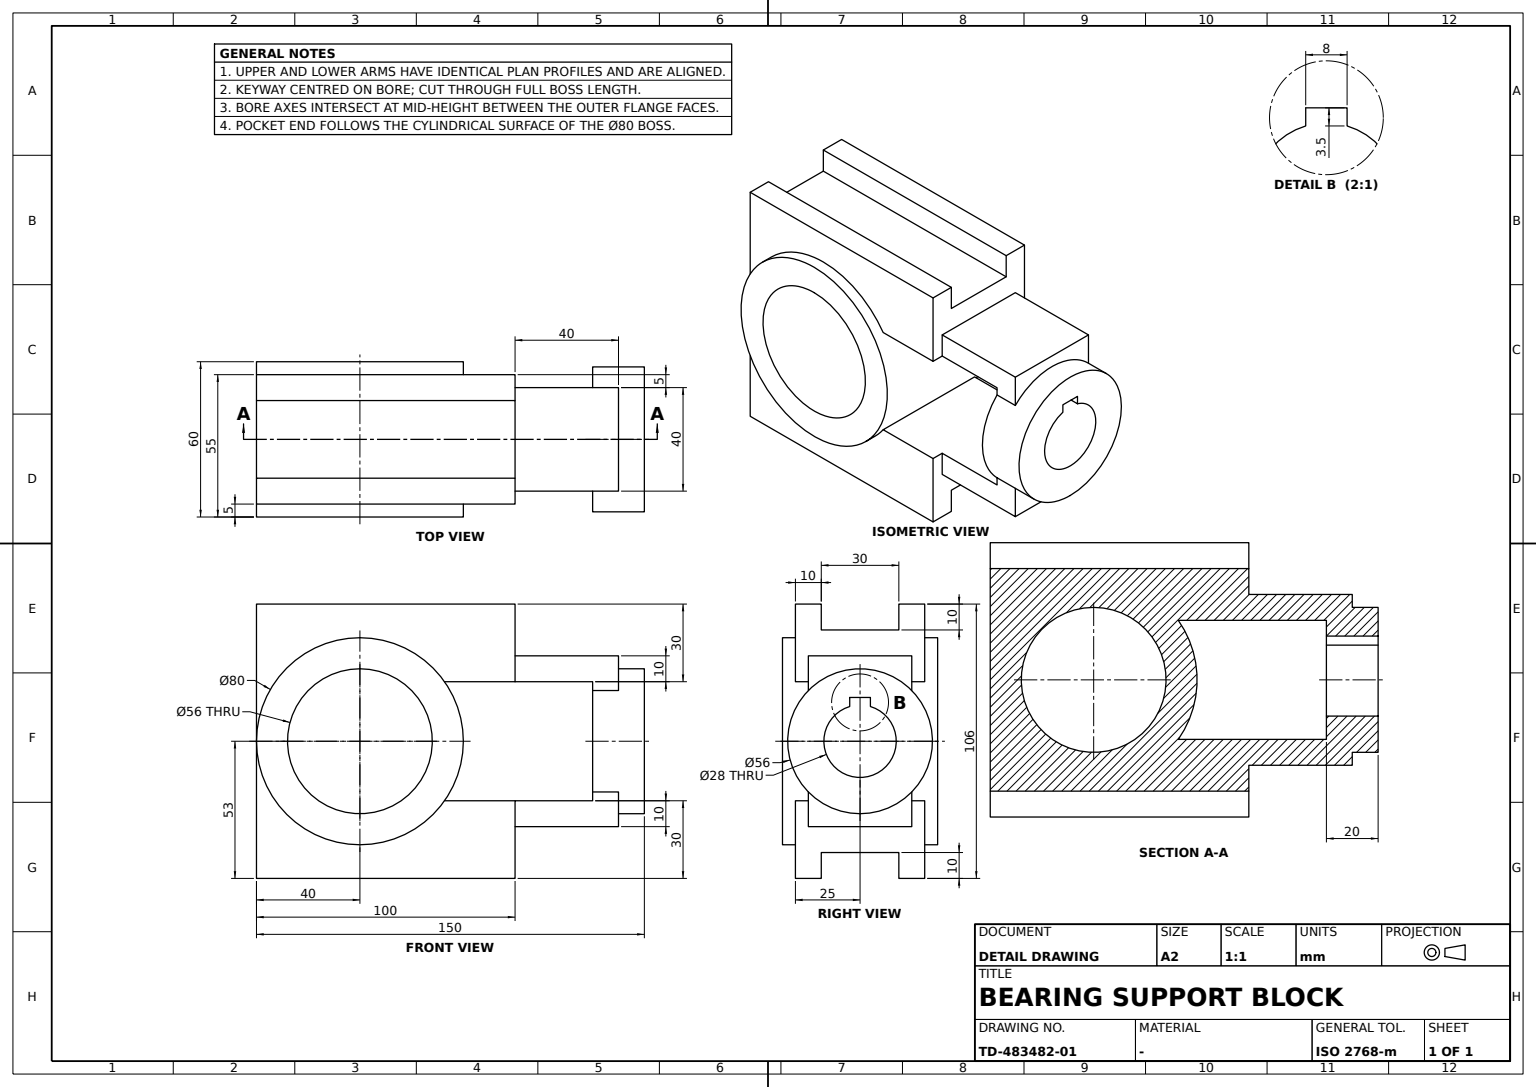
ISO-10303-21;
HEADER;
FILE_DESCRIPTION((''),'2;1');
FILE_NAME('','',(''),(''),'','','');
FILE_SCHEMA(('AUTOMOTIVE_DESIGN'));
ENDSEC;
DATA;
#1=APPLICATION_CONTEXT('');
#2=PRODUCT_CONTEXT('',#1,'mechanical');
#3=PRODUCT('','','',(#2));
#4=PRODUCT_DEFINITION_FORMATION('','',#3);
#5=PRODUCT_DEFINITION_CONTEXT('',#1,'design');
#6=PRODUCT_DEFINITION('','',#4,#5);
#7=PRODUCT_DEFINITION_SHAPE('','',#6);
#8=(LENGTH_UNIT()NAMED_UNIT(*)SI_UNIT(.MILLI.,.METRE.));
#9=(NAMED_UNIT(*)PLANE_ANGLE_UNIT()SI_UNIT($,.RADIAN.));
#10=(NAMED_UNIT(*)SI_UNIT($,.STERADIAN.)SOLID_ANGLE_UNIT());
#11=UNCERTAINTY_MEASURE_WITH_UNIT(LENGTH_MEASURE(0.005),#8,'distance_accuracy_value','');
#12=(GEOMETRIC_REPRESENTATION_CONTEXT(3)GLOBAL_UNCERTAINTY_ASSIGNED_CONTEXT((#11))GLOBAL_UNIT_ASSIGNED_CONTEXT((#8,#9,#10))REPRESENTATION_CONTEXT('',''));
#13=CARTESIAN_POINT('',(40.,-30.,81.));
#14=VERTEX_POINT('',#13);
#15=CARTESIAN_POINT('',(40.,-30.,53.));
#16=DIRECTION('',(0.,1.,0.));
#17=DIRECTION('',(0.,0.,1.));
#18=AXIS2_PLACEMENT_3D('',#15,#16,#17);
#19=CIRCLE('',#18,28.);
#20=EDGE_CURVE('',#14,#14,#19,.T.);
#21=ORIENTED_EDGE('',*,*,#20,.F.);
#22=EDGE_LOOP('',(#21));
#23=FACE_BOUND('',#22,.T.);
#24=CARTESIAN_POINT('',(40.,30.,81.));
#25=VERTEX_POINT('',#24);
#26=CARTESIAN_POINT('',(40.,30.,53.));
#27=AXIS2_PLACEMENT_3D('',#26,#16,#17);
#28=CIRCLE('',#27,28.);
#29=EDGE_CURVE('',#25,#25,#28,.T.);
#30=ORIENTED_EDGE('',*,*,#29,.T.);
#31=EDGE_LOOP('',(#30));
#32=FACE_BOUND('',#31,.T.);
#33=CARTESIAN_POINT('',(40.,29.9,53.));
#34=DIRECTION('',(0.,-1.,0.));
#35=DIRECTION('',(1.,0.,0.));
#36=AXIS2_PLACEMENT_3D('',#33,#34,#35);
#37=CYLINDRICAL_SURFACE('',#36,28.);
#38=ADVANCED_FACE('',(#23,#32),#37,.F.);
#39=CARTESIAN_POINT('',(100.,15.,10.));
#40=VERTEX_POINT('',#39);
#41=CARTESIAN_POINT('',(100.,15.,0.));
#42=VERTEX_POINT('',#41);
#43=CARTESIAN_POINT('',(100.,15.,106.));
#44=DIRECTION('',(0.,0.,-1.));
#45=VECTOR('',#44,1000.);
#46=LINE('',#43,#45);
#47=EDGE_CURVE('',#40,#42,#46,.T.);
#48=ORIENTED_EDGE('',*,*,#47,.F.);
#49=CARTESIAN_POINT('',(0.,15.,10.));
#50=VERTEX_POINT('',#49);
#51=DIRECTION('',(-1.,0.,0.));
#52=VECTOR('',#51,1000.);
#53=LINE('',#39,#52);
#54=EDGE_CURVE('',#40,#50,#53,.T.);
#55=ORIENTED_EDGE('',*,*,#54,.T.);
#56=CARTESIAN_POINT('',(0.,15.,0.));
#57=VERTEX_POINT('',#56);
#58=VECTOR('',#17,1000.);
#59=LINE('',#56,#58);
#60=EDGE_CURVE('',#57,#50,#59,.T.);
#61=ORIENTED_EDGE('',*,*,#60,.F.);
#62=LINE('',#41,#52);
#63=EDGE_CURVE('',#42,#57,#62,.T.);
#64=ORIENTED_EDGE('',*,*,#63,.F.);
#65=EDGE_LOOP('',(#48,#55,#61,#64));
#66=FACE_BOUND('',#65,.T.);
#67=CARTESIAN_POINT('',(100.,15.,96.));
#68=AXIS2_PLACEMENT_3D('',#67,#34,#17);
#69=PLANE('',#68);
#70=ADVANCED_FACE('',(#66),#69,.T.);
#71=CARTESIAN_POINT('',(150.,4.,66.416408));
#72=VERTEX_POINT('',#71);
#73=CARTESIAN_POINT('',(150.,4.,69.916408));
#74=VERTEX_POINT('',#73);
#75=LINE('',#71,#58);
#76=EDGE_CURVE('',#72,#74,#75,.T.);
#77=ORIENTED_EDGE('',*,*,#76,.F.);
#78=CARTESIAN_POINT('',(150.,-4.,66.416408));
#79=VERTEX_POINT('',#78);
#80=CARTESIAN_POINT('',(150.,0.,53.));
#81=AXIS2_PLACEMENT_3D('',#80,#35,#44);
#82=CIRCLE('',#81,14.);
#83=EDGE_CURVE('',#79,#72,#82,.T.);
#84=ORIENTED_EDGE('',*,*,#83,.F.);
#85=CARTESIAN_POINT('',(150.,-4.,69.916408));
#86=VERTEX_POINT('',#85);
#87=LINE('',#85,#45);
#88=EDGE_CURVE('',#86,#79,#87,.T.);
#89=ORIENTED_EDGE('',*,*,#88,.F.);
#90=VECTOR('',#16,1000.);
#91=LINE('',#85,#90);
#92=EDGE_CURVE('',#86,#74,#91,.T.);
#93=ORIENTED_EDGE('',*,*,#92,.T.);
#94=EDGE_LOOP('',(#77,#84,#89,#93));
#95=FACE_BOUND('',#94,.T.);
#96=CARTESIAN_POINT('',(150.,0.,25.));
#97=VERTEX_POINT('',#96);
#98=CIRCLE('',#81,28.);
#99=EDGE_CURVE('',#97,#97,#98,.T.);
#100=ORIENTED_EDGE('',*,*,#99,.T.);
#101=EDGE_LOOP('',(#100));
#102=FACE_BOUND('',#101,.T.);
#103=CARTESIAN_POINT('',(150.,0.,0.));
#104=AXIS2_PLACEMENT_3D('',#103,#35,#16);
#105=PLANE('',#104);
#106=ADVANCED_FACE('',(#95,#102),#105,.T.);
#107=CARTESIAN_POINT('',(40.,30.,93.));
#108=VERTEX_POINT('',#107);
#109=CIRCLE('',#27,40.);
#110=EDGE_CURVE('',#108,#108,#109,.T.);
#111=ORIENTED_EDGE('',*,*,#110,.T.);
#112=EDGE_LOOP('',(#111));
#113=FACE_BOUND('',#112,.T.);
#114=ORIENTED_EDGE('',*,*,#29,.F.);
#115=EDGE_LOOP('',(#114));
#116=FACE_BOUND('',#115,.T.);
#117=CARTESIAN_POINT('',(0.,30.,0.));
#118=AXIS2_PLACEMENT_3D('',#117,#16,#51);
#119=PLANE('',#118);
#120=ADVANCED_FACE('',(#113,#116),#119,.T.);
#121=CARTESIAN_POINT('',(100.,20.,76.));
#122=VERTEX_POINT('',#121);
#123=CARTESIAN_POINT('',(130.,20.,76.));
#124=VERTEX_POINT('',#123);
#125=VECTOR('',#35,1000.);
#126=LINE('',#121,#125);
#127=EDGE_CURVE('',#122,#124,#126,.T.);
#128=ORIENTED_EDGE('',*,*,#127,.F.);
#129=CARTESIAN_POINT('',(100.,20.,86.));
#130=VERTEX_POINT('',#129);
#131=CARTESIAN_POINT('',(100.,20.,106.));
#132=LINE('',#131,#58);
#133=EDGE_CURVE('',#122,#130,#132,.T.);
#134=ORIENTED_EDGE('',*,*,#133,.T.);
#135=CARTESIAN_POINT('',(140.,20.,86.));
#136=VERTEX_POINT('',#135);
#137=LINE('',#129,#125);
#138=EDGE_CURVE('',#130,#136,#137,.T.);
#139=ORIENTED_EDGE('',*,*,#138,.T.);
#140=CARTESIAN_POINT('',(140.,20.,72.595918));
#141=VERTEX_POINT('',#140);
#142=CARTESIAN_POINT('',(140.,20.,76.));
#143=LINE('',#142,#45);
#144=EDGE_CURVE('',#136,#141,#143,.T.);
#145=ORIENTED_EDGE('',*,*,#144,.T.);
#146=CARTESIAN_POINT('',(130.,20.,72.595918));
#147=VERTEX_POINT('',#146);
#148=LINE('',#140,#125);
#149=EDGE_CURVE('',#147,#141,#148,.T.);
#150=ORIENTED_EDGE('',*,*,#149,.F.);
#151=CARTESIAN_POINT('',(130.,20.,30.));
#152=LINE('',#151,#58);
#153=EDGE_CURVE('',#147,#124,#152,.T.);
#154=ORIENTED_EDGE('',*,*,#153,.T.);
#155=EDGE_LOOP('',(#128,#134,#139,#145,#150,#154));
#156=FACE_BOUND('',#155,.T.);
#157=AXIS2_PLACEMENT_3D('',#121,#16,#17);
#158=PLANE('',#157);
#159=ADVANCED_FACE('',(#156),#158,.T.);
#160=CARTESIAN_POINT('',(100.,-20.,86.));
#161=VERTEX_POINT('',#160);
#162=CARTESIAN_POINT('',(140.,-20.,86.));
#163=VERTEX_POINT('',#162);
#164=LINE('',#160,#125);
#165=EDGE_CURVE('',#161,#163,#164,.T.);
#166=ORIENTED_EDGE('',*,*,#165,.F.);
#167=CARTESIAN_POINT('',(100.,-20.,76.));
#168=VERTEX_POINT('',#167);
#169=CARTESIAN_POINT('',(100.,-20.,106.));
#170=LINE('',#169,#45);
#171=EDGE_CURVE('',#161,#168,#170,.T.);
#172=ORIENTED_EDGE('',*,*,#171,.T.);
#173=CARTESIAN_POINT('',(130.,-20.,76.));
#174=VERTEX_POINT('',#173);
#175=LINE('',#167,#125);
#176=EDGE_CURVE('',#168,#174,#175,.T.);
#177=ORIENTED_EDGE('',*,*,#176,.T.);
#178=CARTESIAN_POINT('',(130.,-20.,72.595918));
#179=VERTEX_POINT('',#178);
#180=CARTESIAN_POINT('',(130.,-20.,86.));
#181=LINE('',#180,#58);
#182=EDGE_CURVE('',#179,#174,#181,.T.);
#183=ORIENTED_EDGE('',*,*,#182,.F.);
#184=CARTESIAN_POINT('',(140.,-20.,72.595918));
#185=VERTEX_POINT('',#184);
#186=LINE('',#184,#125);
#187=EDGE_CURVE('',#179,#185,#186,.T.);
#188=ORIENTED_EDGE('',*,*,#187,.T.);
#189=LINE('',#162,#58);
#190=EDGE_CURVE('',#185,#163,#189,.T.);
#191=ORIENTED_EDGE('',*,*,#190,.T.);
#192=EDGE_LOOP('',(#166,#172,#177,#183,#188,#191));
#193=FACE_BOUND('',#192,.T.);
#194=AXIS2_PLACEMENT_3D('',#160,#34,#44);
#195=PLANE('',#194);
#196=ADVANCED_FACE('',(#193),#195,.T.);
#197=CARTESIAN_POINT('',(130.,-4.,69.916408));
#198=VERTEX_POINT('',#197);
#199=CARTESIAN_POINT('',(130.,4.,69.916408));
#200=VERTEX_POINT('',#199);
#201=LINE('',#197,#90);
#202=EDGE_CURVE('',#198,#200,#201,.T.);
#203=ORIENTED_EDGE('',*,*,#202,.T.);
#204=LINE('',#73,#52);
#205=EDGE_CURVE('',#74,#200,#204,.T.);
#206=ORIENTED_EDGE('',*,*,#205,.F.);
#207=ORIENTED_EDGE('',*,*,#92,.F.);
#208=LINE('',#85,#52);
#209=EDGE_CURVE('',#86,#198,#208,.T.);
#210=ORIENTED_EDGE('',*,*,#209,.T.);
#211=EDGE_LOOP('',(#203,#206,#207,#210));
#212=FACE_BOUND('',#211,.T.);
#213=AXIS2_PLACEMENT_3D('',#85,#17,#16);
#214=PLANE('',#213);
#215=ADVANCED_FACE('',(#212),#214,.F.);
#216=CARTESIAN_POINT('',(0.,-25.,106.));
#217=VERTEX_POINT('',#216);
#218=CARTESIAN_POINT('',(100.,-25.,106.));
#219=VERTEX_POINT('',#218);
#220=LINE('',#216,#125);
#221=EDGE_CURVE('',#217,#219,#220,.T.);
#222=ORIENTED_EDGE('',*,*,#221,.T.);
#223=CARTESIAN_POINT('',(100.,-15.,106.));
#224=VERTEX_POINT('',#223);
#225=CARTESIAN_POINT('',(100.,0.,106.));
#226=LINE('',#225,#90);
#227=EDGE_CURVE('',#219,#224,#226,.T.);
#228=ORIENTED_EDGE('',*,*,#227,.T.);
#229=CARTESIAN_POINT('',(0.,-15.,106.));
#230=VERTEX_POINT('',#229);
#231=LINE('',#229,#52);
#232=EDGE_CURVE('',#224,#230,#231,.T.);
#233=ORIENTED_EDGE('',*,*,#232,.T.);
#234=CARTESIAN_POINT('',(0.,0.,106.));
#235=LINE('',#234,#90);
#236=EDGE_CURVE('',#217,#230,#235,.T.);
#237=ORIENTED_EDGE('',*,*,#236,.F.);
#238=EDGE_LOOP('',(#222,#228,#233,#237));
#239=FACE_BOUND('',#238,.T.);
#240=AXIS2_PLACEMENT_3D('',#234,#17,#35);
#241=PLANE('',#240);
#242=ADVANCED_FACE('',(#239),#241,.T.);
#243=CARTESIAN_POINT('',(130.,4.,66.416408));
#244=VERTEX_POINT('',#243);
#245=LINE('',#243,#58);
#246=EDGE_CURVE('',#244,#200,#245,.T.);
#247=ORIENTED_EDGE('',*,*,#246,.F.);
#248=LINE('',#71,#125);
#249=EDGE_CURVE('',#72,#244,#248,.F.);
#250=ORIENTED_EDGE('',*,*,#249,.F.);
#251=ORIENTED_EDGE('',*,*,#76,.T.);
#252=ORIENTED_EDGE('',*,*,#205,.T.);
#253=EDGE_LOOP('',(#247,#250,#251,#252));
#254=FACE_BOUND('',#253,.T.);
#255=AXIS2_PLACEMENT_3D('',#71,#34,#17);
#256=PLANE('',#255);
#257=ADVANCED_FACE('',(#254),#256,.T.);
#258=CARTESIAN_POINT('',(100.,25.,30.));
#259=VERTEX_POINT('',#258);
#260=CARTESIAN_POINT('',(100.,25.,0.));
#261=VERTEX_POINT('',#260);
#262=LINE('',#260,#45);
#263=EDGE_CURVE('',#259,#261,#262,.T.);
#264=ORIENTED_EDGE('',*,*,#263,.T.);
#265=CARTESIAN_POINT('',(0.,25.,0.));
#266=VERTEX_POINT('',#265);
#267=LINE('',#265,#52);
#268=EDGE_CURVE('',#261,#266,#267,.T.);
#269=ORIENTED_EDGE('',*,*,#268,.T.);
#270=CARTESIAN_POINT('',(0.,25.,53.));
#271=VERTEX_POINT('',#270);
#272=LINE('',#265,#58);
#273=EDGE_CURVE('',#266,#271,#272,.T.);
#274=ORIENTED_EDGE('',*,*,#273,.T.);
#275=CARTESIAN_POINT('',(72.726136,25.,30.));
#276=VERTEX_POINT('',#275);
#277=CARTESIAN_POINT('',(40.,25.,53.));
#278=AXIS2_PLACEMENT_3D('',#277,#16,#17);
#279=CIRCLE('',#278,40.);
#280=EDGE_CURVE('',#276,#271,#279,.T.);
#281=ORIENTED_EDGE('',*,*,#280,.F.);
#282=CARTESIAN_POINT('',(0.,25.,30.));
#283=LINE('',#282,#125);
#284=EDGE_CURVE('',#276,#259,#283,.T.);
#285=ORIENTED_EDGE('',*,*,#284,.T.);
#286=EDGE_LOOP('',(#264,#269,#274,#281,#285));
#287=FACE_BOUND('',#286,.T.);
#288=AXIS2_PLACEMENT_3D('',#265,#16,#51);
#289=PLANE('',#288);
#290=ADVANCED_FACE('',(#287),#289,.T.);
#291=CARTESIAN_POINT('',(140.,0.,86.));
#292=LINE('',#291,#90);
#293=EDGE_CURVE('',#163,#136,#292,.T.);
#294=ORIENTED_EDGE('',*,*,#293,.T.);
#295=ORIENTED_EDGE('',*,*,#138,.F.);
#296=CARTESIAN_POINT('',(100.,0.,86.));
#297=LINE('',#296,#90);
#298=EDGE_CURVE('',#161,#130,#297,.T.);
#299=ORIENTED_EDGE('',*,*,#298,.F.);
#300=ORIENTED_EDGE('',*,*,#165,.T.);
#301=EDGE_LOOP('',(#294,#295,#299,#300));
#302=FACE_BOUND('',#301,.T.);
#303=AXIS2_PLACEMENT_3D('',#160,#44,#16);
#304=PLANE('',#303);
#305=ADVANCED_FACE('',(#302),#304,.F.);
#306=CARTESIAN_POINT('',(0.,25.,106.));
#307=VERTEX_POINT('',#306);
#308=CARTESIAN_POINT('',(100.,25.,106.));
#309=VERTEX_POINT('',#308);
#310=LINE('',#306,#125);
#311=EDGE_CURVE('',#307,#309,#310,.T.);
#312=ORIENTED_EDGE('',*,*,#311,.F.);
#313=CARTESIAN_POINT('',(0.,15.,106.));
#314=VERTEX_POINT('',#313);
#315=EDGE_CURVE('',#314,#307,#235,.T.);
#316=ORIENTED_EDGE('',*,*,#315,.F.);
#317=VERTEX_POINT('',#43);
#318=LINE('',#43,#52);
#319=EDGE_CURVE('',#317,#314,#318,.T.);
#320=ORIENTED_EDGE('',*,*,#319,.F.);
#321=EDGE_CURVE('',#317,#309,#226,.T.);
#322=ORIENTED_EDGE('',*,*,#321,.T.);
#323=EDGE_LOOP('',(#312,#316,#320,#322));
#324=FACE_BOUND('',#323,.T.);
#325=ADVANCED_FACE('',(#324),#241,.T.);
#326=ORIENTED_EDGE('',*,*,#249,.T.);
#327=CARTESIAN_POINT('',(130.,-4.,66.416408));
#328=VERTEX_POINT('',#327);
#329=CARTESIAN_POINT('',(130.,0.,53.));
#330=AXIS2_PLACEMENT_3D('',#329,#35,#44);
#331=CIRCLE('',#330,14.);
#332=EDGE_CURVE('',#328,#244,#331,.T.);
#333=ORIENTED_EDGE('',*,*,#332,.F.);
#334=LINE('',#78,#125);
#335=EDGE_CURVE('',#79,#328,#334,.F.);
#336=ORIENTED_EDGE('',*,*,#335,.F.);
#337=ORIENTED_EDGE('',*,*,#83,.T.);
#338=EDGE_LOOP('',(#326,#333,#336,#337));
#339=FACE_BOUND('',#338,.T.);
#340=CARTESIAN_POINT('',(140.,0.,53.));
#341=AXIS2_PLACEMENT_3D('',#340,#35,#16);
#342=CYLINDRICAL_SURFACE('',#341,14.);
#343=ADVANCED_FACE('',(#339),#342,.F.);
#344=ORIENTED_EDGE('',*,*,#88,.T.);
#345=ORIENTED_EDGE('',*,*,#335,.T.);
#346=LINE('',#197,#45);
#347=EDGE_CURVE('',#198,#328,#346,.T.);
#348=ORIENTED_EDGE('',*,*,#347,.F.);
#349=ORIENTED_EDGE('',*,*,#209,.F.);
#350=EDGE_LOOP('',(#344,#345,#348,#349));
#351=FACE_BOUND('',#350,.T.);
#352=AXIS2_PLACEMENT_3D('',#85,#16,#44);
#353=PLANE('',#352);
#354=ADVANCED_FACE('',(#351),#353,.T.);
#355=CARTESIAN_POINT('',(100.,25.,76.));
#356=VERTEX_POINT('',#355);
#357=CARTESIAN_POINT('',(100.,0.,76.));
#358=LINE('',#357,#90);
#359=EDGE_CURVE('',#122,#356,#358,.T.);
#360=ORIENTED_EDGE('',*,*,#359,.F.);
#361=ORIENTED_EDGE('',*,*,#127,.T.);
#362=CARTESIAN_POINT('',(130.,0.,76.));
#363=VECTOR('',#34,1000.);
#364=LINE('',#362,#363);
#365=EDGE_CURVE('',#124,#174,#364,.T.);
#366=ORIENTED_EDGE('',*,*,#365,.T.);
#367=ORIENTED_EDGE('',*,*,#176,.F.);
#368=CARTESIAN_POINT('',(100.,-25.,76.));
#369=VERTEX_POINT('',#368);
#370=EDGE_CURVE('',#369,#168,#358,.T.);
#371=ORIENTED_EDGE('',*,*,#370,.F.);
#372=CARTESIAN_POINT('',(72.726136,-25.,76.));
#373=VERTEX_POINT('',#372);
#374=CARTESIAN_POINT('',(0.,-25.,76.));
#375=LINE('',#374,#52);
#376=EDGE_CURVE('',#369,#373,#375,.T.);
#377=ORIENTED_EDGE('',*,*,#376,.T.);
#378=CARTESIAN_POINT('',(72.726136,25.,76.));
#379=VERTEX_POINT('',#378);
#380=LINE('',#372,#90);
#381=EDGE_CURVE('',#373,#379,#380,.T.);
#382=ORIENTED_EDGE('',*,*,#381,.T.);
#383=CARTESIAN_POINT('',(0.,25.,76.));
#384=LINE('',#383,#52);
#385=EDGE_CURVE('',#356,#379,#384,.T.);
#386=ORIENTED_EDGE('',*,*,#385,.F.);
#387=EDGE_LOOP('',(#360,#361,#366,#367,#371,#377,#382,#386));
#388=FACE_BOUND('',#387,.T.);
#389=AXIS2_PLACEMENT_3D('',#357,#44,#51);
#390=PLANE('',#389);
#391=ADVANCED_FACE('',(#388),#390,.T.);
#392=ORIENTED_EDGE('',*,*,#221,.F.);
#393=CARTESIAN_POINT('',(0.,-25.,53.));
#394=VERTEX_POINT('',#393);
#395=CARTESIAN_POINT('',(0.,-25.,0.));
#396=LINE('',#395,#58);
#397=EDGE_CURVE('',#394,#217,#396,.T.);
#398=ORIENTED_EDGE('',*,*,#397,.F.);
#399=CARTESIAN_POINT('',(40.,-25.,53.));
#400=AXIS2_PLACEMENT_3D('',#399,#16,#17);
#401=CIRCLE('',#400,40.);
#402=EDGE_CURVE('',#394,#373,#401,.T.);
#403=ORIENTED_EDGE('',*,*,#402,.T.);
#404=ORIENTED_EDGE('',*,*,#376,.F.);
#405=CARTESIAN_POINT('',(100.,-25.,0.));
#406=LINE('',#405,#45);
#407=EDGE_CURVE('',#219,#369,#406,.T.);
#408=ORIENTED_EDGE('',*,*,#407,.F.);
#409=EDGE_LOOP('',(#392,#398,#403,#404,#408));
#410=FACE_BOUND('',#409,.T.);
#411=AXIS2_PLACEMENT_3D('',#395,#16,#51);
#412=PLANE('',#411);
#413=ADVANCED_FACE('',(#410),#412,.F.);
#414=ORIENTED_EDGE('',*,*,#268,.F.);
#415=CARTESIAN_POINT('',(100.,0.,0.));
#416=LINE('',#415,#90);
#417=EDGE_CURVE('',#42,#261,#416,.T.);
#418=ORIENTED_EDGE('',*,*,#417,.F.);
#419=ORIENTED_EDGE('',*,*,#63,.T.);
#420=CARTESIAN_POINT('',(0.,0.,0.));
#421=LINE('',#420,#90);
#422=EDGE_CURVE('',#57,#266,#421,.T.);
#423=ORIENTED_EDGE('',*,*,#422,.T.);
#424=EDGE_LOOP('',(#414,#418,#419,#423));
#425=FACE_BOUND('',#424,.T.);
#426=AXIS2_PLACEMENT_3D('',#415,#44,#51);
#427=PLANE('',#426);
#428=ADVANCED_FACE('',(#425),#427,.T.);
#429=EDGE_CURVE('',#271,#307,#272,.T.);
#430=ORIENTED_EDGE('',*,*,#429,.F.);
#431=ORIENTED_EDGE('',*,*,#273,.F.);
#432=ORIENTED_EDGE('',*,*,#422,.F.);
#433=ORIENTED_EDGE('',*,*,#60,.T.);
#434=CARTESIAN_POINT('',(0.,-15.,10.));
#435=VERTEX_POINT('',#434);
#436=CARTESIAN_POINT('',(0.,0.,10.));
#437=LINE('',#436,#363);
#438=EDGE_CURVE('',#50,#435,#437,.T.);
#439=ORIENTED_EDGE('',*,*,#438,.T.);
#440=CARTESIAN_POINT('',(0.,-15.,0.));
#441=VERTEX_POINT('',#440);
#442=LINE('',#229,#58);
#443=EDGE_CURVE('',#441,#435,#442,.T.);
#444=ORIENTED_EDGE('',*,*,#443,.F.);
#445=VERTEX_POINT('',#395);
#446=EDGE_CURVE('',#445,#441,#421,.T.);
#447=ORIENTED_EDGE('',*,*,#446,.F.);
#448=EDGE_CURVE('',#445,#394,#396,.T.);
#449=ORIENTED_EDGE('',*,*,#448,.T.);
#450=ORIENTED_EDGE('',*,*,#397,.T.);
#451=ORIENTED_EDGE('',*,*,#236,.T.);
#452=CARTESIAN_POINT('',(0.,-15.,96.));
#453=VERTEX_POINT('',#452);
#454=LINE('',#440,#45);
#455=EDGE_CURVE('',#230,#453,#454,.T.);
#456=ORIENTED_EDGE('',*,*,#455,.T.);
#457=CARTESIAN_POINT('',(0.,15.,96.));
#458=VERTEX_POINT('',#457);
#459=CARTESIAN_POINT('',(0.,0.,96.));
#460=LINE('',#459,#363);
#461=EDGE_CURVE('',#458,#453,#460,.T.);
#462=ORIENTED_EDGE('',*,*,#461,.F.);
#463=LINE('',#457,#45);
#464=EDGE_CURVE('',#314,#458,#463,.T.);
#465=ORIENTED_EDGE('',*,*,#464,.F.);
#466=ORIENTED_EDGE('',*,*,#315,.T.);
#467=EDGE_LOOP('',(#430,#431,#432,#433,#439,#444,#447,#449,#450,#451,#456,#462,#465,#466));
#468=FACE_BOUND('',#467,.T.);
#469=AXIS2_PLACEMENT_3D('',#420,#51,#17);
#470=PLANE('',#469);
#471=ADVANCED_FACE('',(#468),#470,.T.);
#472=ORIENTED_EDGE('',*,*,#110,.F.);
#473=EDGE_LOOP('',(#472));
#474=FACE_BOUND('',#473,.T.);
#475=CARTESIAN_POINT('',(40.,-30.,93.));
#476=VERTEX_POINT('',#475);
#477=CIRCLE('',#18,40.);
#478=EDGE_CURVE('',#476,#476,#477,.T.);
#479=ORIENTED_EDGE('',*,*,#478,.T.);
#480=EDGE_LOOP('',(#479));
#481=FACE_BOUND('',#480,.T.);
#482=ORIENTED_EDGE('',*,*,#381,.F.);
#483=ORIENTED_EDGE('',*,*,#402,.F.);
#484=CARTESIAN_POINT('',(72.726136,-25.,30.));
#485=VERTEX_POINT('',#484);
#486=EDGE_CURVE('',#485,#394,#401,.T.);
#487=ORIENTED_EDGE('',*,*,#486,.F.);
#488=LINE('',#484,#90);
#489=EDGE_CURVE('',#485,#276,#488,.T.);
#490=ORIENTED_EDGE('',*,*,#489,.T.);
#491=ORIENTED_EDGE('',*,*,#280,.T.);
#492=EDGE_CURVE('',#271,#379,#279,.T.);
#493=ORIENTED_EDGE('',*,*,#492,.T.);
#494=EDGE_LOOP('',(#482,#483,#487,#490,#491,#493));
#495=FACE_BOUND('',#494,.T.);
#496=CARTESIAN_POINT('',(40.,0.,53.));
#497=AXIS2_PLACEMENT_3D('',#496,#16,#51);
#498=CYLINDRICAL_SURFACE('',#497,40.);
#499=ADVANCED_FACE('',(#474,#481,#495),#498,.T.);
#500=CARTESIAN_POINT('',(100.,-25.,30.));
#501=VERTEX_POINT('',#500);
#502=CARTESIAN_POINT('',(0.,-25.,30.));
#503=LINE('',#502,#125);
#504=EDGE_CURVE('',#485,#501,#503,.T.);
#505=ORIENTED_EDGE('',*,*,#504,.F.);
#506=ORIENTED_EDGE('',*,*,#486,.T.);
#507=ORIENTED_EDGE('',*,*,#448,.F.);
#508=VERTEX_POINT('',#405);
#509=LINE('',#395,#52);
#510=EDGE_CURVE('',#508,#445,#509,.T.);
#511=ORIENTED_EDGE('',*,*,#510,.F.);
#512=EDGE_CURVE('',#501,#508,#406,.T.);
#513=ORIENTED_EDGE('',*,*,#512,.F.);
#514=EDGE_LOOP('',(#505,#506,#507,#511,#513));
#515=FACE_BOUND('',#514,.T.);
#516=ADVANCED_FACE('',(#515),#412,.F.);
#517=ORIENTED_EDGE('',*,*,#144,.F.);
#518=ORIENTED_EDGE('',*,*,#293,.F.);
#519=ORIENTED_EDGE('',*,*,#190,.F.);
#520=AXIS2_PLACEMENT_3D('',#340,#35,#44);
#521=CIRCLE('',#520,28.);
#522=EDGE_CURVE('',#141,#185,#521,.T.);
#523=ORIENTED_EDGE('',*,*,#522,.F.);
#524=EDGE_LOOP('',(#517,#518,#519,#523));
#525=FACE_BOUND('',#524,.T.);
#526=CARTESIAN_POINT('',(140.,0.,0.));
#527=AXIS2_PLACEMENT_3D('',#526,#35,#16);
#528=PLANE('',#527);
#529=ADVANCED_FACE('',(#525),#528,.T.);
#530=ORIENTED_EDGE('',*,*,#438,.F.);
#531=ORIENTED_EDGE('',*,*,#54,.F.);
#532=CARTESIAN_POINT('',(100.,-15.,10.));
#533=VERTEX_POINT('',#532);
#534=LINE('',#39,#363);
#535=EDGE_CURVE('',#40,#533,#534,.T.);
#536=ORIENTED_EDGE('',*,*,#535,.T.);
#537=LINE('',#532,#52);
#538=EDGE_CURVE('',#533,#435,#537,.T.);
#539=ORIENTED_EDGE('',*,*,#538,.T.);
#540=EDGE_LOOP('',(#530,#531,#536,#539));
#541=FACE_BOUND('',#540,.T.);
#542=AXIS2_PLACEMENT_3D('',#39,#44,#34);
#543=PLANE('',#542);
#544=ADVANCED_FACE('',(#541),#543,.T.);
#545=ORIENTED_EDGE('',*,*,#365,.F.);
#546=ORIENTED_EDGE('',*,*,#153,.F.);
#547=CARTESIAN_POINT('',(130.,20.,33.404082));
#548=VERTEX_POINT('',#547);
#549=CIRCLE('',#330,28.);
#550=EDGE_CURVE('',#548,#147,#549,.T.);
#551=ORIENTED_EDGE('',*,*,#550,.F.);
#552=VERTEX_POINT('',#151);
#553=EDGE_CURVE('',#552,#548,#152,.T.);
#554=ORIENTED_EDGE('',*,*,#553,.F.);
#555=CARTESIAN_POINT('',(130.,-20.,30.));
#556=VERTEX_POINT('',#555);
#557=LINE('',#151,#363);
#558=EDGE_CURVE('',#552,#556,#557,.T.);
#559=ORIENTED_EDGE('',*,*,#558,.T.);
#560=CARTESIAN_POINT('',(130.,-20.,33.404082));
#561=VERTEX_POINT('',#560);
#562=EDGE_CURVE('',#556,#561,#181,.T.);
#563=ORIENTED_EDGE('',*,*,#562,.T.);
#564=EDGE_CURVE('',#179,#561,#549,.T.);
#565=ORIENTED_EDGE('',*,*,#564,.F.);
#566=ORIENTED_EDGE('',*,*,#182,.T.);
#567=EDGE_LOOP('',(#545,#546,#551,#554,#559,#563,#565,#566));
#568=FACE_BOUND('',#567,.T.);
#569=ORIENTED_EDGE('',*,*,#246,.T.);
#570=ORIENTED_EDGE('',*,*,#202,.F.);
#571=ORIENTED_EDGE('',*,*,#347,.T.);
#572=ORIENTED_EDGE('',*,*,#332,.T.);
#573=EDGE_LOOP('',(#569,#570,#571,#572));
#574=FACE_BOUND('',#573,.T.);
#575=AXIS2_PLACEMENT_3D('',#151,#35,#17);
#576=PLANE('',#575);
#577=ADVANCED_FACE('',(#568,#574),#576,.F.);
#578=CARTESIAN_POINT('',(100.,-20.,20.));
#579=VERTEX_POINT('',#578);
#580=CARTESIAN_POINT('',(100.,20.,20.));
#581=VERTEX_POINT('',#580);
#582=CARTESIAN_POINT('',(100.,0.,20.));
#583=LINE('',#582,#90);
#584=EDGE_CURVE('',#579,#581,#583,.T.);
#585=ORIENTED_EDGE('',*,*,#584,.F.);
#586=CARTESIAN_POINT('',(100.,-20.,30.));
#587=VERTEX_POINT('',#586);
#588=LINE('',#160,#58);
#589=EDGE_CURVE('',#579,#587,#588,.T.);
#590=ORIENTED_EDGE('',*,*,#589,.T.);
#591=CARTESIAN_POINT('',(100.,0.,30.));
#592=LINE('',#591,#90);
#593=EDGE_CURVE('',#501,#587,#592,.T.);
#594=ORIENTED_EDGE('',*,*,#593,.F.);
#595=ORIENTED_EDGE('',*,*,#512,.T.);
#596=CARTESIAN_POINT('',(100.,-15.,0.));
#597=VERTEX_POINT('',#596);
#598=EDGE_CURVE('',#508,#597,#416,.T.);
#599=ORIENTED_EDGE('',*,*,#598,.T.);
#600=LINE('',#223,#58);
#601=EDGE_CURVE('',#597,#533,#600,.T.);
#602=ORIENTED_EDGE('',*,*,#601,.T.);
#603=ORIENTED_EDGE('',*,*,#535,.F.);
#604=ORIENTED_EDGE('',*,*,#47,.T.);
#605=ORIENTED_EDGE('',*,*,#417,.T.);
#606=ORIENTED_EDGE('',*,*,#263,.F.);
#607=CARTESIAN_POINT('',(100.,20.,30.));
#608=VERTEX_POINT('',#607);
#609=EDGE_CURVE('',#608,#259,#592,.T.);
#610=ORIENTED_EDGE('',*,*,#609,.F.);
#611=LINE('',#121,#45);
#612=EDGE_CURVE('',#608,#581,#611,.T.);
#613=ORIENTED_EDGE('',*,*,#612,.T.);
#614=EDGE_LOOP('',(#585,#590,#594,#595,#599,#602,#603,#604,#605,#606,#610,#613));
#615=FACE_BOUND('',#614,.T.);
#616=AXIS2_PLACEMENT_3D('',#225,#35,#44);
#617=PLANE('',#616);
#618=ADVANCED_FACE('',(#615),#617,.T.);
#619=ORIENTED_EDGE('',*,*,#538,.F.);
#620=ORIENTED_EDGE('',*,*,#601,.F.);
#621=LINE('',#596,#52);
#622=EDGE_CURVE('',#597,#441,#621,.T.);
#623=ORIENTED_EDGE('',*,*,#622,.T.);
#624=ORIENTED_EDGE('',*,*,#443,.T.);
#625=EDGE_LOOP('',(#619,#620,#623,#624));
#626=FACE_BOUND('',#625,.T.);
#627=AXIS2_PLACEMENT_3D('',#223,#16,#44);
#628=PLANE('',#627);
#629=ADVANCED_FACE('',(#626),#628,.T.);
#630=ORIENTED_EDGE('',*,*,#298,.T.);
#631=ORIENTED_EDGE('',*,*,#133,.F.);
#632=ORIENTED_EDGE('',*,*,#359,.T.);
#633=EDGE_CURVE('',#309,#356,#262,.T.);
#634=ORIENTED_EDGE('',*,*,#633,.F.);
#635=ORIENTED_EDGE('',*,*,#321,.F.);
#636=VERTEX_POINT('',#67);
#637=LINE('',#67,#58);
#638=EDGE_CURVE('',#636,#317,#637,.T.);
#639=ORIENTED_EDGE('',*,*,#638,.F.);
#640=CARTESIAN_POINT('',(100.,-15.,96.));
#641=VERTEX_POINT('',#640);
#642=LINE('',#67,#363);
#643=EDGE_CURVE('',#636,#641,#642,.T.);
#644=ORIENTED_EDGE('',*,*,#643,.T.);
#645=LINE('',#223,#45);
#646=EDGE_CURVE('',#224,#641,#645,.T.);
#647=ORIENTED_EDGE('',*,*,#646,.F.);
#648=ORIENTED_EDGE('',*,*,#227,.F.);
#649=ORIENTED_EDGE('',*,*,#407,.T.);
#650=ORIENTED_EDGE('',*,*,#370,.T.);
#651=ORIENTED_EDGE('',*,*,#171,.F.);
#652=EDGE_LOOP('',(#630,#631,#632,#634,#635,#639,#644,#647,#648,#649,#650,#651));
#653=FACE_BOUND('',#652,.T.);
#654=ADVANCED_FACE('',(#653),#617,.T.);
#655=ORIENTED_EDGE('',*,*,#646,.T.);
#656=LINE('',#640,#52);
#657=EDGE_CURVE('',#641,#453,#656,.T.);
#658=ORIENTED_EDGE('',*,*,#657,.T.);
#659=ORIENTED_EDGE('',*,*,#455,.F.);
#660=ORIENTED_EDGE('',*,*,#232,.F.);
#661=EDGE_LOOP('',(#655,#658,#659,#660));
#662=FACE_BOUND('',#661,.T.);
#663=ADVANCED_FACE('',(#662),#628,.T.);
#664=ORIENTED_EDGE('',*,*,#99,.F.);
#665=EDGE_LOOP('',(#664));
#666=FACE_BOUND('',#665,.T.);
#667=ORIENTED_EDGE('',*,*,#187,.F.);
#668=ORIENTED_EDGE('',*,*,#564,.T.);
#669=CARTESIAN_POINT('',(140.,-20.,33.404082));
#670=VERTEX_POINT('',#669);
#671=LINE('',#669,#125);
#672=EDGE_CURVE('',#670,#561,#671,.F.);
#673=ORIENTED_EDGE('',*,*,#672,.F.);
#674=CARTESIAN_POINT('',(140.,20.,33.404082));
#675=VERTEX_POINT('',#674);
#676=EDGE_CURVE('',#670,#675,#521,.T.);
#677=ORIENTED_EDGE('',*,*,#676,.T.);
#678=LINE('',#674,#125);
#679=EDGE_CURVE('',#675,#548,#678,.F.);
#680=ORIENTED_EDGE('',*,*,#679,.T.);
#681=ORIENTED_EDGE('',*,*,#550,.T.);
#682=ORIENTED_EDGE('',*,*,#149,.T.);
#683=ORIENTED_EDGE('',*,*,#522,.T.);
#684=EDGE_LOOP('',(#667,#668,#673,#677,#680,#681,#682,#683));
#685=FACE_BOUND('',#684,.T.);
#686=CYLINDRICAL_SURFACE('',#341,28.);
#687=ADVANCED_FACE('',(#666,#685),#686,.T.);
#688=CARTESIAN_POINT('',(70.,-20.,30.));
#689=LINE('',#688,#125);
#690=EDGE_CURVE('',#587,#556,#689,.T.);
#691=ORIENTED_EDGE('',*,*,#690,.F.);
#692=ORIENTED_EDGE('',*,*,#589,.F.);
#693=CARTESIAN_POINT('',(140.,-20.,20.));
#694=VERTEX_POINT('',#693);
#695=LINE('',#578,#125);
#696=EDGE_CURVE('',#579,#694,#695,.T.);
#697=ORIENTED_EDGE('',*,*,#696,.T.);
#698=EDGE_CURVE('',#694,#670,#189,.T.);
#699=ORIENTED_EDGE('',*,*,#698,.T.);
#700=ORIENTED_EDGE('',*,*,#672,.T.);
#701=ORIENTED_EDGE('',*,*,#562,.F.);
#702=EDGE_LOOP('',(#691,#692,#697,#699,#700,#701));
#703=FACE_BOUND('',#702,.T.);
#704=ADVANCED_FACE('',(#703),#195,.T.);
#705=ORIENTED_EDGE('',*,*,#478,.F.);
#706=EDGE_LOOP('',(#705));
#707=FACE_BOUND('',#706,.T.);
#708=ORIENTED_EDGE('',*,*,#20,.T.);
#709=EDGE_LOOP('',(#708));
#710=FACE_BOUND('',#709,.T.);
#711=CARTESIAN_POINT('',(0.,-30.,0.));
#712=AXIS2_PLACEMENT_3D('',#711,#16,#51);
#713=PLANE('',#712);
#714=ADVANCED_FACE('',(#707,#710),#713,.F.);
#715=ORIENTED_EDGE('',*,*,#638,.T.);
#716=ORIENTED_EDGE('',*,*,#319,.T.);
#717=ORIENTED_EDGE('',*,*,#464,.T.);
#718=LINE('',#67,#52);
#719=EDGE_CURVE('',#636,#458,#718,.T.);
#720=ORIENTED_EDGE('',*,*,#719,.F.);
#721=EDGE_LOOP('',(#715,#716,#717,#720));
#722=FACE_BOUND('',#721,.T.);
#723=ADVANCED_FACE('',(#722),#69,.T.);
#724=LINE('',#607,#125);
#725=EDGE_CURVE('',#608,#552,#724,.T.);
#726=ORIENTED_EDGE('',*,*,#725,.T.);
#727=ORIENTED_EDGE('',*,*,#553,.T.);
#728=ORIENTED_EDGE('',*,*,#679,.F.);
#729=CARTESIAN_POINT('',(140.,20.,20.));
#730=VERTEX_POINT('',#729);
#731=EDGE_CURVE('',#675,#730,#143,.T.);
#732=ORIENTED_EDGE('',*,*,#731,.T.);
#733=LINE('',#580,#125);
#734=EDGE_CURVE('',#581,#730,#733,.T.);
#735=ORIENTED_EDGE('',*,*,#734,.F.);
#736=ORIENTED_EDGE('',*,*,#612,.F.);
#737=EDGE_LOOP('',(#726,#727,#728,#732,#735,#736));
#738=FACE_BOUND('',#737,.T.);
#739=ADVANCED_FACE('',(#738),#158,.T.);
#740=ORIENTED_EDGE('',*,*,#584,.T.);
#741=ORIENTED_EDGE('',*,*,#734,.T.);
#742=CARTESIAN_POINT('',(140.,0.,20.));
#743=LINE('',#742,#90);
#744=EDGE_CURVE('',#694,#730,#743,.T.);
#745=ORIENTED_EDGE('',*,*,#744,.F.);
#746=ORIENTED_EDGE('',*,*,#696,.F.);
#747=EDGE_LOOP('',(#740,#741,#745,#746));
#748=FACE_BOUND('',#747,.T.);
#749=AXIS2_PLACEMENT_3D('',#578,#44,#16);
#750=PLANE('',#749);
#751=ADVANCED_FACE('',(#748),#750,.T.);
#752=ORIENTED_EDGE('',*,*,#489,.F.);
#753=ORIENTED_EDGE('',*,*,#504,.T.);
#754=ORIENTED_EDGE('',*,*,#593,.T.);
#755=ORIENTED_EDGE('',*,*,#690,.T.);
#756=ORIENTED_EDGE('',*,*,#558,.F.);
#757=ORIENTED_EDGE('',*,*,#725,.F.);
#758=ORIENTED_EDGE('',*,*,#609,.T.);
#759=ORIENTED_EDGE('',*,*,#284,.F.);
#760=EDGE_LOOP('',(#752,#753,#754,#755,#756,#757,#758,#759));
#761=FACE_BOUND('',#760,.T.);
#762=CARTESIAN_POINT('',(70.,0.,30.));
#763=AXIS2_PLACEMENT_3D('',#762,#17,#35);
#764=PLANE('',#763);
#765=ADVANCED_FACE('',(#761),#764,.T.);
#766=ORIENTED_EDGE('',*,*,#429,.T.);
#767=ORIENTED_EDGE('',*,*,#311,.T.);
#768=ORIENTED_EDGE('',*,*,#633,.T.);
#769=ORIENTED_EDGE('',*,*,#385,.T.);
#770=ORIENTED_EDGE('',*,*,#492,.F.);
#771=EDGE_LOOP('',(#766,#767,#768,#769,#770));
#772=FACE_BOUND('',#771,.T.);
#773=ADVANCED_FACE('',(#772),#289,.T.);
#774=ORIENTED_EDGE('',*,*,#510,.T.);
#775=ORIENTED_EDGE('',*,*,#446,.T.);
#776=ORIENTED_EDGE('',*,*,#622,.F.);
#777=ORIENTED_EDGE('',*,*,#598,.F.);
#778=EDGE_LOOP('',(#774,#775,#776,#777));
#779=FACE_BOUND('',#778,.T.);
#780=ADVANCED_FACE('',(#779),#427,.T.);
#781=ORIENTED_EDGE('',*,*,#744,.T.);
#782=ORIENTED_EDGE('',*,*,#731,.F.);
#783=ORIENTED_EDGE('',*,*,#676,.F.);
#784=ORIENTED_EDGE('',*,*,#698,.F.);
#785=EDGE_LOOP('',(#781,#782,#783,#784));
#786=FACE_BOUND('',#785,.T.);
#787=ADVANCED_FACE('',(#786),#528,.T.);
#788=ORIENTED_EDGE('',*,*,#643,.F.);
#789=ORIENTED_EDGE('',*,*,#719,.T.);
#790=ORIENTED_EDGE('',*,*,#461,.T.);
#791=ORIENTED_EDGE('',*,*,#657,.F.);
#792=EDGE_LOOP('',(#788,#789,#790,#791));
#793=FACE_BOUND('',#792,.T.);
#794=AXIS2_PLACEMENT_3D('',#67,#44,#34);
#795=PLANE('',#794);
#796=ADVANCED_FACE('',(#793),#795,.F.);
#797=CLOSED_SHELL('',(#38,#70,#106,#120,#159,#196,#215,#242,#257,#290,#305,#325,#343,#354,#391,#413,#428,#471,#499,#516,#529,#544,#577,#618,#629,#654,#663,#687,#704,#714,#723,#739,#751,#765,#773,#780,#787,#796));
#798=MANIFOLD_SOLID_BREP('',#797);
#799=ADVANCED_BREP_SHAPE_REPRESENTATION('',(#798),#12);
#800=SHAPE_DEFINITION_REPRESENTATION(#7,#799);
ENDSEC;
END-ISO-10303-21;
